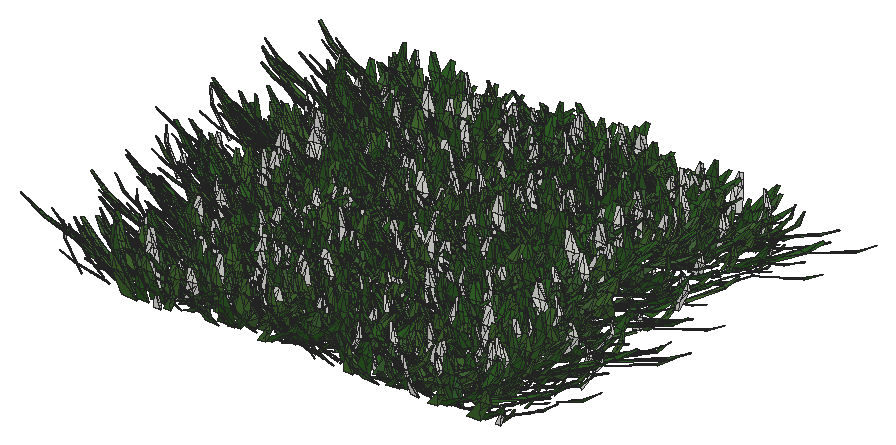
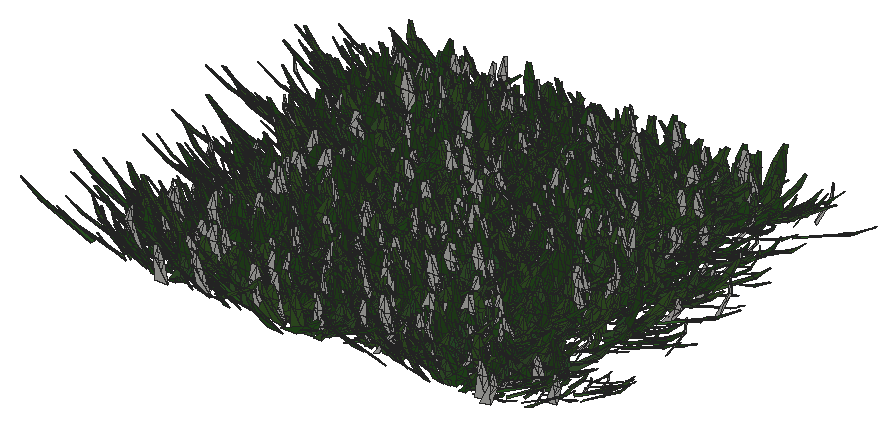
# SketchUp Ruby script. Lengths in inches.
U = 1.inch
M = Sketchup.active_model
def pt(a) = Geom::Point3d.new(a.map { |v| v * U })
def face(e, loops, mat)
  f = e.add_face(loops[0].map { |a| pt(a) })
  loops[1..].each { |l| e.add_face(l.map { |a| pt(a) }).erase! }
  f.material = f.back_material = mat if mat
  f
end
# faces: each face lists its corners as indices into pts; further lists are holes
def faces(e, pts, list, mat = nil) = list.each { |f| face(e, (f[0].is_a?(Array) ? f : [f]).map { |l| l.map { |i| pts[i] } }, mat) }
# xy, xz, yz: faces in a plane at the given z, y or x. An outline is a flat list of corners, or four numbers for a rectangle; further outlines are holes
def ring(l) = l.size == 4 ? [[l[0], l[1]], [l[2], l[1]], [l[2], l[3]], [l[0], l[3]]] : l.each_slice(2).to_a
def flat(e, list, mat, &to3) = list.each { |f| face(e, (f[0].is_a?(Array) ? f : [f]).map { |l| ring(l).map { |u, v| to3.(u, v) } }, mat) }
def xy(e, z, list, mat = nil) = flat(e, list, mat) { |x, y| [x, y, z] }
def xz(e, y, list, mat = nil) = flat(e, list, mat) { |x, z| [x, y, z] }
def yz(e, x, list, mat = nil) = flat(e, list, mat) { |y, z| [x, y, z] }
def lines(e, pts, list) = list.each { |a, b| e.add_line(pt(pts[a]), pt(pts[b])) }
# prism: a flat outline (further loops are holes) pulled along v
def prism(e, loops, v, mat = nil)
  f = face(e, loops, mat); d = Geom::Vector3d.new(v.map { |x| x * U })
  f.pushpull(f.normal.samedirection?(d) ? d.length : -d.length)
end
def box(e, o, s, mat = nil) = prism(e, [[o, [o[0] + s[0], o[1], o[2]], [o[0] + s[0], o[1] + s[1], o[2]], [o[0], o[1] + s[1], o[2]]]], [0, 0, s[2]], mat)
def at(x, y, z, deg = 0) = Geom::Transformation.translation(pt([x, y, z])) * Geom::Transformation.rotation(ORIGIN, Z_AXIS, deg.degrees)
def axes(o, x, y, z) = Geom::Transformation.new([*x, 0, *y, 0, *z, 0, *pt(o).to_a, 1])
def part(name) = M.definitions.add(name)
# library, detail: a bought-in or finely detailed component or shape, given as its bounding box
def library(name, o, s) = part(name).tap { |d| box(d.entities, o, s) }
def detail(e, o, s) = box(e.add_group.entities, o, s)
def put(e, d, t, mat = nil) = e.add_instance(d, t).tap { |i| i.material = mat if mat }
def group(e, t, mat = nil) = e.add_group.tap { |g| g.transformation = t; g.material = mat if mat }.entities
root = M.entities
M.materials.add("Material10").color = [48, 100, 38]
M.materials.add("Material3").color = [68, 110, 58]
M.materials.add("Material4").color = [48, 90, 38]
M.materials.add("Material5").color = [68, 110, 48]
M.materials.add("Material6").color = [48, 90, 48]
M.materials.add("Material7").color = [58, 110, 58]
M.materials.add("Material8").color = [58, 90, 38]
M.materials.add("Material9").color = [68, 100, 58]
c1 = part("grass00")
p = [[-0.6875,0.15,0],[-0.56,0.08,5.52],[-0.04,0.03,2.76],[0.48,-0.02,0],[0.35,-0.02,5.52],[-0.1,-0.14,5.52],
  [-0.12,0.65,8.37],[-0.42,0.65,8.37]]
faces(c1.entities,p,[[0,1,2,3],[3,2,4],[1,5,2],[5,4,2],[1,6,5],[4,5,6],[7,6,1]])
c2 = part("Group16\#1")
put(c2.entities,c1,axes([1.44,-0.61,-0.01],[0.05352,0.12609,0],[-0.10704,0.04543,0.07239],[0.06664,-0.02828,0.11628]),"Material6")
put(c2.entities,c1,axes([0.76,-0.15,-0.01],[0.04676,0.24062,0],[-0.23162,0.04501,0.06642],[0.0652,-0.01267,0.23595]),"Material3")
put(c2.entities,c1,axes([0.79,0.01,-0.01],[-0.00606,0.34651,0],[-0.34381,-0.00602,0.0432],[0.04319,0.00076,0.34386]))
put(c2.entities,c1,axes([1,0.23,-0.01],[-0.07192,0.31144,0],[-0.28722,-0.06632,0.1236],[0.12043,0.02781,0.29478]),"Material5")
put(c2.entities,c1,axes([1.66,0.77,-0.01],[-0.13828,0.29651,0],[-0.21551,-0.1005,0.22471],[0.20365,0.09498,0.23779]),"Material10")
put(c2.entities,c1,axes([0.6875,0.52,-0.01],[-0.18126,0.24051,0],[-0.22746,-0.17142,0.09788],[0.07817,0.05891,0.28481]),"Material5")
put(c2.entities,c1,axes([0.68,0.78,-0.01],[-0.215,0.18688,0],[-0.12385,-0.14248,0.21334],[0.13995,0.16101,0.18878]),"Material3")
put(c2.entities,c1,axes([0.56,1,-0.01],[-0.13756,0.07624,0],[-0.06159,-0.11112,0.0927],[0.04494,0.08108,0.12705]),"Material5")
put(c2.entities,c1,axes([0.2,0.64,-0.01],[-0.23729,0.07254,0],[-0.05711,-0.18681,0.153],[0.04473,0.14632,0.19535]),"Material10")
put(c2.entities,c1,axes([0.0625,0.72,-0.01],[-0.28874,0.02525,0],[-0.02179,-0.24916,0.14647],[0.01276,0.14591,0.25012]),"Material3")
put(c2.entities,c1,axes([-0.08,0.62,-0.01],[-0.34089,-0.04187,0],[0.03255,-0.26504,0.216],[-0.02633,0.21439,0.26703]),"Material10")
put(c2.entities,c1,axes([-0.34,0.98,-0.01],[-0.14314,-0.0493,0],[0.04397,-0.12769,0.06843],[-0.02228,0.0647,0.13505]),"Material10")
put(c2.entities,c1,axes([-0.87,1.45,-0.01],[-0.23488,-0.14114,0],[0.13761,-0.22901,0.06087],[-0.03135,0.05217,0.26717]))
put(c2.entities,c1,axes([-0.72,0.77,-0.01],[-0.14208,-0.13251,0],[0.07209,-0.0773,0.16301],[-0.11118,0.11922,0.1057]),"Material10")
put(c2.entities,c1,axes([-0.62,0.43,-0.01],[-0.14845,-0.21203,0],[0.18654,-0.13061,0.12304],[-0.10079,0.07057,0.22772]),"Material3")
put(c2.entities,c1,axes([-0.68,0.29,-0.01],[-0.13639,-0.32136,0],[0.31723,-0.13464,0.05579],[-0.05136,0.0218,0.34462]),"Material4")
put(c2.entities,c1,axes([-0.64,0.125,-0.01],[-0.0458,-0.23569,0],[0.22124,-0.043,0.08276],[-0.08124,0.01579,0.22538]),"Material7")
put(c2.entities,c1,axes([-1.6,-0.03,-0.01],[0.00576,-0.32897,0],[0.27526,0.00482,0.18018],[-0.18015,-0.00315,0.2753]),"Material5")
put(c2.entities,c1,axes([-1.36,-0.31,-0.01],[0.05718,-0.24765,0],[0.18172,0.04196,0.17267],[-0.16825,-0.03885,0.1865]),"Material10")
put(c2.entities,c1,axes([-1.54,-0.72,-0.01],[0.06537,-0.14017,0],[0.13555,0.06321,0.03939],[-0.0357,-0.01665,0.14956]))
put(c2.entities,c1,axes([-1.19,-0.9,-0.01],[0.09597,-0.12735,0],[0.11214,0.08451,0.07557],[-0.06035,-0.04548,0.14042]),"Material9")
put(c2.entities,c1,axes([-0.47,-0.54,-0.01],[0.11588,-0.10072,0],[0.0618,0.0711,0.12124],[-0.07953,-0.0915,0.0942]))
put(c2.entities,c1,axes([-0.47,-0.84,-0.01],[0.11927,-0.0661,0],[0.06603,0.11913,0.00646],[-0.00313,-0.00565,0.13621]),"Material5")
put(c2.entities,c1,axes([-0.38,-1.24,-0.01],[0.28037,-0.08571,0],[0.0618,0.20215,0.20315],[-0.05939,-0.19428,0.21139]),"Material9")
put(c2.entities,c1,axes([-0.06,-0.66,-0.01],[0.22719,-0.01987,0],[0.01247,0.14255,0.17758],[-0.01547,-0.17691,0.1431]),"Material8")
put(c2.entities,c1,axes([0.11,-0.89,-0.01],[0.14882,0.01828,0],[-0.01058,0.08611,0.12229],[0.01491,-0.12138,0.08676]),"Material6")
put(c2.entities,c1,axes([0.25,-0.72,-0.01],[0.20481,0.07053,0],[-0.06206,0.18022,0.10291],[0.03351,-0.0973,0.1906]),"Material6")
put(c2.entities,c1,axes([0.85,-1.42,-0.01],[0.16481,0.09904,0],[-0.09472,0.15762,0.05616],[0.02893,-0.04814,0.18389]),"Material5")
put(c2.entities,c1,axes([1.01,-1.09,-0.01],[0.21858,0.20385,0],[-0.17495,0.1876,0.15339],[0.10462,-0.11218,0.25652]),"Material10")
put(c2.entities,c1,axes([1.01,-0.71,-0.01],[0.08733,0.12473,0],[-0.06445,0.04512,0.13037],[0.1068,-0.07477,0.07867]),"Material6")
c3 = part("Group15\#1")
put(c3.entities,c2,at(0,0,0))
c4 = part("3darcstudiotree_grass00\#1")
put(c4.entities,c3,at(0,0,0))
put(root,c4,axes([1060.01,968.44,0],[3.81538,0.13844,0],[-0.69714,1.20077,-0.0224],[-0.01503,0.02589,1.41716]))
put(root,c4,axes([1060.61,966.34,0],[3.87873,-0.1816,0],[0.87965,1.17427,-0.05648],[0.04872,0.06503,1.39957]))
put(root,c4,axes([1060.62,949.85,0],[2.2908,0.71526,0],[-3.14647,0.62983,-0.01526],[-0.09231,0.01848,1.9517]))
put(root,c4,axes([1060.87,957.6,0],[1.88546,0.82083,0],[-4.0871,0.58676,-0.0451],[-0.25686,0.03688,1.93445]))
put(root,c4,axes([1064,960.65,0],[-3.85189,-0.43073,0],[1.56903,-0.87695,-0.00732],[0.02092,-0.01169,1.68082]))
put(root,c4,axes([1063.95,942.66,0],[-1.50152,-0.9142,0],[4.09435,-0.4203,-0.04381],[0.2556,-0.02624,1.74465]))
put(root,c4,axes([1064.63,951.69,0],[-0.92252,-0.87304,0],[4.75689,-0.31416,-0.01354],[0.0811,-0.00536,1.90468]))
put(root,c4,axes([1063.46,971.5,0],[4.15823,-0.14638,0],[0.56684,1.00637,-0.04526],[0.04452,0.07905,1.7925]))
put(root,c4,axes([1065.13,934.82,0],[-1.25145,-1.20565,0],[3.82205,-0.24795,-0.03225],[0.20024,-0.01299,1.58326]))
put(root,c4,axes([1064.48,958.88,0],[-3.10495,0.65805,0],[-2.73218,-0.80572,-0.0209],[-0.07578,-0.02235,1.48072]))
put(root,c4,axes([1063.8,933.42,0],[0.14781,1.06815,0],[-4.11052,0.03555,-0.02489],[-0.18669,0.00161,1.9295]))
put(root,c4,axes([1063.73,948.06,0],[4.00072,0.7254,0],[-2.30793,0.79554,-0.01189],[-0.04272,0.01473,1.50367]))
put(root,c4,axes([1064.75,958.07,0],[-2.74027,0.72148,0],[-3.68495,-0.87475,-0.01749],[-0.07151,-0.01698,1.7911]))
put(root,c4,axes([1065.1,945.05,0],[-2.75544,0.79472,0],[-3.06036,-0.66317,-0.04719],[-0.18345,-0.03975,1.30223]))
put(root,c4,axes([1065.82,968.08,0],[1.11217,-0.96649,0],[4.59277,0.33032,-0.0144],[0.08373,0.00602,1.80693]))
put(root,c4,axes([1065.92,954.83,0],[-4.93169,0.08818,0],[-0.36054,-1.26027,-0.06114],[-0.024,-0.08388,1.73764]))
put(root,c4,axes([1064.06,952.93,0],[3.76135,0.71254,0],[-2.83931,0.93675,-0.0181],[-0.05013,0.01654,1.34745]))
put(root,c4,axes([1064.44,964.01,0],[0.92537,1.06658,0],[-3.52867,0.19134,-0.00976],[-0.0687,0.00373,1.62508]))
put(root,c4,axes([1065.98,936.2,0],[-4.59841,0.23812,0],[-1.05246,-1.27026,-0.05761],[-0.06188,-0.07469,1.71741]))
put(root,c4,axes([1065.1,950.4375,0],[3.52248,-0.74116,0],[2.46477,0.73213,-0.04982],[0.1917,0.05694,1.4295]))
put(root,c4,axes([1065.57,956.52,0],[-2.75303,1.02553,0],[-3.67007,-0.61577,-0.03945],[-0.19029,-0.03193,1.6047]))
put(root,c4,axes([1066.68,938.42,0],[0.13208,-1.10378,0],[4.58182,0.03427,-0.01737],[0.09381,0.0007,1.54781]))
put(root,c4,axes([1065.45,972.2,0],[3.94098,0.32291,0],[-1.45311,1.10842,-0.04711],[-0.07836,0.05977,1.55738]))
put(root,c4,axes([1067.3,946.65,0],[-4.05461,-0.34542,0],[1.65205,-1.21201,-0.06303],[0.10229,-0.07504,1.61067]))
put(root,c4,axes([1066.19,939.92,0],[-0.37634,1.08622,0],[-3.78806,-0.08203,-0.04948],[-0.29529,-0.00639,1.42361]))
put(root,c4,axes([1065.71,943.77,0],[1.93194,0.81354,0],[-3.84457,0.57061,-0.05173],[-0.21974,0.03261,1.38038]))
put(root,c4,axes([1067.08,969.37,0],[2.66553,-1.02305,0],[4.32772,0.70474,-0.04483],[0.19345,0.0315,1.66248]))
put(root,c4,axes([1067.12,966.35,0],[-4.37352,0.6514,0],[-2.31701,-0.97227,-0.00882],[-0.02275,-0.00955,1.42641]))
put(root,c4,axes([1066.53,940.98,0],[4.99102,-0.01521,0],[0.04604,0.94447,-0.04731],[0.00388,0.07956,1.58849]))
put(root,c4,axes([1067.67,964.9375,0],[3.89455,0.04164,0],[-0.19515,1.14083,-0.05798],[-0.01392,0.08139,1.60438]))
put(root,c4,axes([1067.37,961.9,0],[2.5974,0.75785,0],[-3.87592,0.83025,-0.05975],[-0.19783,0.04238,1.3909]))
put(root,c4,axes([1070.43,954.99,0],[-4.50466,-0.2627,0],[0.84333,-0.90382,-0.01564],[0.02098,-0.02248,1.3694]))
put(root,c4,axes([1071.07,951.4,0],[-4.10148,-0.37644,0],[1.4137,-0.96268,-0.02574],[0.04791,-0.03263,1.38465]))
put(root,c4,axes([1070.94,948.83,0],[-4.28392,0.00118,0],[-0.00439,-0.99985,-0.04481],[-0.00034,-0.07634,1.70362]))
put(root,c4,axes([1071.18,963.31,0],[-4.02766,-0.18324,0],[0.7232,-0.9935,-0.02729],[0.03622,-0.04975,1.8715]))
put(root,c4,axes([1071.04,965.58,0],[1.16692,-1.18724,0],[4.2577,0.26155,-0.05295],[0.37072,0.02277,1.97565]))
put(root,c4,axes([1071.97,959.11,0],[-4.78558,-0.30533,0],[0.89073,-0.87254,-0.00096],[0.00166,-0.00163,1.58162]))
put(root,c4,axes([1071.53,962.42,0],[1.62332,-1.0011,0],[4.766,0.48301,-0.03495],[0.18538,0.01879,1.83937]))
put(root,c4,axes([1072.25,941.04,0],[-4.37321,-0.34262,0],[1.17174,-0.93477,-0.00157],[0.00264,-0.00211,1.37913]))
put(root,c4,axes([1071.75,960.11,0],[0.5215,-1.25098,0],[3.70627,0.09657,-0.02929],[0.19507,0.00508,1.55926]))
put(root,c4,axes([1072.1875,935.32,0],[-1.52927,-0.99373,0],[4.10162,-0.3945,-0.0371],[0.24735,-0.02379,1.96201]))
put(root,c4,axes([1071.96,970.28,0],[-2.5925,0.65112,0],[-2.57682,-0.64124,-0.04592],[-0.2048,-0.05096,1.42994]))
put(root,c4,axes([1070.98,952.76,0],[2.46517,0.89808,0],[-3.36918,0.57801,-0.0512],[-0.22975,0.03942,1.38975]))
put(root,c4,axes([1071.74,946.98,0],[-1.95791,0.95694,0],[-3.80128,-0.48609,-0.05082],[-0.22925,-0.02932,1.35221]))
put(root,c4,axes([1070.95,945.78,0],[3.4935,0.9356,0],[-3.37227,0.78699,-0.04297],[-0.21601,0.05041,1.98261]))
put(root,c4,axes([1072.5625,949.54,0],[-3.83195,0.74101,0],[-2.84787,-0.92045,-0.05181],[-0.15821,-0.05114,1.45196]))
put(root,c4,axes([1072.74,968.71,0],[1.45199,-1.1226,0],[3.82197,0.30896,-0.02554],[0.13596,0.01099,1.40467]))
put(root,c4,axes([1072.63,958.05,0],[0.21484,-1.19151,0],[3.62833,0.04089,-0.03915],[0.33615,0.00379,1.95085]))
put(root,c4,axes([1072.78,944.46,0],[-4.05301,0.5506,0],[-2.43371,-1.11967,-0.04664],[-0.11424,-0.05256,1.63424]))
put(root,c4,axes([1072.64,956.5625,0],[2.22271,-0.98365,0],[3.97274,0.56106,-0.05349],[0.32137,0.04539,1.96798]))
put(root,c4,axes([1071.54,971.14,0],[2.83397,0.77998,0],[-3.02687,0.68736,-0.01914],[-0.0787,0.01787,1.41957]))
put(root,c4,axes([1071.36,936.42,0],[1.59207,1.04289,0],[-4.49774,0.42914,-0.00597],[-0.03376,0.00322,1.82255]))
put(root,c4,axes([1071.99,933.84,0],[3.98575,0.27966,0],[-0.97946,0.87245,-0.00495],[-0.0082,0.00731,1.38942]))
put(root,c4,axes([1072.27,966.23,0],[4.21135,-0.01817,0],[0.08044,1.16521,-0.0287],[0.00337,0.04884,1.98369]))
put(root,c4,axes([1072.75,939.42,0],[-2.028,0.74895,0],[-3.60661,-0.61038,-0.00267],[-0.01315,-0.00223,1.62102]))
put(root,c4,axes([1073.56,942.1,0],[3.07423,-0.81379,0],[3.32943,0.78609,-0.05261],[0.18555,0.04381,1.38839]))
put(root,c4,axes([1072.82,937.74,0],[3.5941,0.56914,0],[-2.69156,1.06232,-0.01012],[-0.02733,0.01079,1.58691]))
put(root,c4,axes([1075.71,940.98,0],[-0.91152,-0.89442,0],[3.63132,-0.23129,-0.03395],[0.21582,-0.01375,1.53644]))
put(root,c4,axes([1076.09,943.5,0],[-0.47866,-0.98426,0],[5.08014,-0.15441,-0.04217],[0.1851,-0.00563,1.41426]))
put(root,c4,axes([1076.28,954.85,0],[-3.99249,-0.2843,0],[1.19862,-1.05202,-0.03955],[0.07734,-0.06788,1.95202]))
put(root,c4,axes([1075.46,947.38,0],[4.25304,-0.27501,0],[1.24647,1.20478,-0.04841],[0.06924,0.06692,1.77682]))
put(root,c4,axes([1075.74,959.03,0],[3.55406,-0.41539,0],[2.08359,1.1142,-0.04906],[0.12364,0.06612,1.82977]))
put(root,c4,axes([1077.04,936.3125,0],[-0.93715,-1.08339,0],[4.95712,-0.268,-0.05631],[0.2396,-0.01295,1.37991]))
put(root,c4,axes([1077.33,945.36,0],[-3.14134,-0.50366,0],[2.13341,-0.83163,-0.01822],[0.06361,-0.0248,1.59761]))
put(root,c4,axes([1077.07,938.9375,0],[-3.94175,0.51659,0],[-1.67373,-0.7982,-0.02232],[-0.07314,-0.03488,1.59039]))
put(root,c4,axes([1075.57,948.76,0],[1.62757,0.88807,0],[-4.34169,0.49732,-0.00338],[-0.01586,0.00182,1.53978]))
put(root,c4,axes([1076.37,968.32,0],[4.57989,-0.16103,0],[0.69599,1.23718,-0.01318],[0.01167,0.02075,1.98636]))
put(root,c4,axes([1077.74,951.39,0],[1.79397,-1.16047,0],[4.15779,0.40172,-0.011],[0.05477,0.00529,1.48653]))
put(root,c4,axes([1078.22,935.36,0],[-3.09464,-0.54466,0],[2.39537,-0.85062,-0.03828],[0.16794,-0.05964,1.98208]))
put(root,c4,axes([1076.89,957.33,0],[0.16957,1.15455,0],[-4.45398,0.04088,-0.05084],[-0.31058,0.00285,1.70302]))
put(root,c4,axes([1077.39,961.91,0],[3.46351,-0.6215,0],[2.10035,0.73155,-0.02763],[0.09487,0.03304,1.3256]))
put(root,c4,axes([1078.47,956.5,0],[-1.3865,-0.85758,0],[4.31936,-0.43646,-0.05241],[0.27908,-0.0282,1.67241]))
put(root,c4,axes([1078.63,965.44,0],[-4.39937,-0.11992,0],[0.44419,-1.01847,-0.05296],[0.03633,-0.08329,1.62079]))
put(root,c4,axes([1079.33,938.4,0],[-1.76031,-0.79386,0],[4.32977,-0.60005,-0.00731],[0.04086,-0.00566,1.97847]))
put(root,c4,axes([1079.32,969.55,0],[-2.83446,-0.91757,0],[3.42874,-0.66198,-0.00917],[0.043,-0.0083,1.60374]))
put(root,c4,axes([1078.99,963.69,0],[-0.96511,-1.1714,0],[4.02104,-0.20706,-0.02826],[0.17189,-0.00885,1.59374]))
put(root,c4,axes([1078.17,966.53,0],[-2.51846,0.95711,0],[-4.14801,-0.68217,-0.04701],[-0.20561,-0.03381,1.62457]))
put(root,c4,axes([1079.36,950.15,0],[-3.64421,0.19897,0],[-0.82865,-0.94858,-0.01018],[-0.01217,-0.01393,1.35975]))
put(root,c4,axes([1078.29,942.02,0],[4.36646,0.14498,0],[-0.67462,1.26988,-0.05242],[-0.04036,0.07596,1.87281]))
put(root,c4,axes([1079.25,971.55,0],[3.61828,-0.3087,0],[1.22458,0.89709,-0.02189],[0.0555,0.04066,1.86062]))
put(root,c4,axes([1079.38,952.58,0],[-0.33218,0.92371,0],[-3.73108,-0.08386,-0.0349],[-0.21038,-0.00473,1.41691]))
put(root,c4,axes([1079.45,961.08,0],[3.6543,-0.06929,0],[0.34871,1.14948,-0.06006],[0.02412,0.07952,1.53056]))
put(root,c4,axes([1079.95,972.55,0],[2.4776,1.07425,0],[-3.76626,0.5429,-0.02249],[-0.11657,0.0168,1.62577]))
put(root,c4,axes([1081.93,961,0],[1.28704,-1.14477,0],[4.41434,0.31018,-0.04021],[0.23445,0.01647,1.73573]))
put(root,c4,axes([1082.32,966.49,0],[-3.66743,0.44114,0],[-1.9663,-1.02167,-0.05656],[-0.13362,-0.06943,1.54444]))
put(root,c4,axes([1082.53,971.34,0],[-3.63818,0.44085,0],[-1.59896,-0.82474,-0.04774],[-0.15109,-0.07793,1.66266]))
put(root,c4,axes([1082.95,936.69,0],[-3.07397,-0.63014,0],[2.5257,-0.77005,-0.04795],[0.16981,-0.05177,1.39039]))
put(root,c4,axes([1081.92,938.9,0],[3.59272,-0.42375,0],[1.98946,1.05421,-0.02435],[0.06043,0.03202,1.69455]))
put(root,c4,axes([1083.11,964.9,0],[-2.26382,-1.02381,0],[3.25832,-0.45029,-0.04183],[0.23401,-0.03234,1.48723]))
put(root,c4,axes([1083.21,949.46,0],[-1.57651,-1.12747,0],[4.0703,-0.35571,-0.03865],[0.26242,-0.02293,1.9383]))
put(root,c4,axes([1081.78,963.1,0],[1.17301,1.14331,0],[-4.44463,0.28501,-0.04684],[-0.2246,0.0144,1.41954]))
put(root,c4,axes([1081.97,955.125,0],[4.31123,0.22817,0],[-0.83721,0.9887,-0.03259],[-0.04316,0.05097,1.61556]))
put(root,c4,axes([1081.96,969.97,0],[3.06774,1.03902,0],[-3.08129,0.5686,-0.03251],[-0.17928,0.03308,1.64081]))
put(root,c4,axes([1084.33,962.35,0],[-2.08621,-0.85991,0],[3.58173,-0.54309,-0.01057],[0.06396,-0.0097,1.85267]))
put(root,c4,axes([1083.97,951.53,0],[-4.18093,0.10999,0],[-0.54376,-1.29184,-0.00853],[-0.00476,-0.01131,1.7318]))
put(root,c4,axes([1084.74,941.4375,0],[-3.42299,-0.52038,0],[2.6642,-1.0953,-0.06276],[0.1523,-0.06261,1.49667]))
put(root,c4,axes([1082.96,938.17,0],[3.25907,0.53746,0],[-2.27195,0.86105,-0.03997],[-0.15705,0.05952,1.84008]))
put(root,c4,axes([1084.98,943.54,0],[-2.53551,-0.66282,0],[3.06498,-0.73279,-0.03327],[0.11879,-0.0284,1.30962]))
put(root,c4,axes([1083.78,959.47,0],[-1.21767,0.90066,0],[-3.71776,-0.31415,-0.04196],[-0.263,-0.02222,1.62262]))
put(root,c4,axes([1085.06,946.81,0],[-4.32463,-0.20055,0],[0.81802,-1.10246,-0.00704],[0.00853,-0.0115,1.86241]))
put(root,c4,axes([1083.54,955.625,0],[-0.94156,1.16657,0],[-3.85079,-0.19425,-0.00527],[-0.04036,-0.00204,1.91768]))
put(root,c4,axes([1083.86,953.26,0],[-1.89095,0.77708,0],[-4.00997,-0.60986,-0.02284],[-0.10942,-0.01664,1.64481]))
put(root,c4,axes([1084.66,967.76,0],[-3.52622,0.53949,0],[-2.34194,-0.95671,-0.04749],[-0.11586,-0.04733,1.3106]))
put(root,c4,axes([1084.31,941.9375,0],[-0.72165,1.07172,0],[-4.22626,-0.17786,-0.04712],[-0.23093,-0.00972,1.33133]))
put(root,c4,axes([1083.87,945.625,0],[1.97727,0.77994,0],[-4.30152,0.68157,-0.01772],[-0.06482,0.01027,1.37883]))
put(root,c4,axes([1085.28,934.88,0],[3.9848,-0.55599,0],[2.03989,0.91374,-0.03495],[0.12387,0.05549,1.90256]))
put(root,c4,axes([1085.09,972.32,0],[-0.75919,1.1846,0],[-4.72482,-0.18925,-0.01053],[-0.05452,-0.00218,1.56894]))
put(root,c4,axes([1085.86,948.05,0],[-2.69032,0.86465,0],[-3.81847,-0.74256,-0.01031],[-0.04487,-0.00873,1.66779]))
put(root,c4,axes([1085.23,957.34,0],[4.37586,0.6715,0],[-2.05906,0.83863,-0.0354],[-0.14622,0.05955,1.94218]))
put(root,c4,axes([1087.94,971.52,0],[3.53194,-0.86434,0],[3.34252,0.85365,-0.00616],[0.02391,0.00611,1.65812]))
put(root,c4,axes([1087.54,942.53,0],[-1.22084,1.17012,0],[-4.22614,-0.27558,-0.04083],[-0.27889,-0.01819,1.92702]))
put(root,c4,axes([1088.77,956.5625,0],[2.5391,-0.86121,0],[4.09888,0.75529,-0.00987],[0.04755,0.00876,1.9048]))
put(root,c4,axes([1088.11,952.86,0],[4.20042,-0.44882,0],[1.64886,0.96446,-0.01454],[0.02841,0.01662,1.30369]))
put(root,c4,axes([1089.15,967.04,0],[-3.69839,0.06543,0],[-0.3293,-1.16339,-0.01026],[-0.00422,-0.01493,1.70108]))
put(root,c4,axes([1088.65,962.53,0],[2.45158,-0.94892,0],[4.05066,0.65407,-0.0579],[0.29835,0.04817,1.84885]))
put(root,c4,axes([1089.03,951.41,0],[-3.62062,0.56511,0],[-2.64905,-1.06077,-0.02972],[-0.08176,-0.03274,1.62371]))
put(root,c4,axes([1088.37,960.49,0],[4.94305,-0.26827,0],[1.01972,1.17431,-0.03342],[0.04517,0.05201,1.91382]))
put(root,c4,axes([1088.93,934.53,0],[5.06338,0.28931,0],[-0.91613,1.00212,-0.00333],[-0.00395,0.00432,1.36941]))
put(root,c4,axes([1090.74,939.61,0],[-3.99538,-0.04123,0],[0.20618,-1.24865,-0.05407],[0.01202,-0.0728,1.68402]))
put(root,c4,axes([1089.16,936.07,0],[2.5961,0.65731,0],[-3.59247,0.8868,-0.04002],[-0.16483,0.04069,1.82631]))
put(root,c4,axes([1090.21,949.96,0],[-3.34956,0.74843,0],[-3.0511,-0.85344,-0.02716],[-0.08391,-0.02347,1.32671]))
put(root,c4,axes([1091.4375,948.29,0],[-2.33326,-1.15563,0],[4.19034,-0.52878,-0.02075],[0.1057,-0.01334,1.67433]))
put(root,c4,axes([1090.15,967.84,0],[3.85684,-0.72833,0],[2.27457,0.7528,-0.01203],[0.05895,0.01951,1.91781]))
put(root,c4,axes([1091.38,940.99,0],[-4.81633,-0.15482,0],[0.50253,-0.97708,-0.03967],[0.03663,-0.07121,1.78282]))
put(root,c4,axes([1091.26,959.49,0],[-4.3189,0.23802,0],[-0.87038,-0.98708,-0.01188],[-0.02021,-0.02292,1.99665]))
put(root,c4,axes([1090.68,954.46,0],[3.261,-0.91173,0],[3.2122,0.71807,-0.03435],[0.17461,0.03903,1.83666]))
put(root,c4,axes([1089.98,963.71,0],[0.9409,1.10722,0],[-4.02636,0.21385,-0.01067],[-0.07425,0.00394,1.82972]))
put(root,c4,axes([1091.71,945.78,0],[-4.23033,0.08475,0],[-0.4056,-1.2654,-0.02116],[-0.00955,-0.02979,1.79229]))
put(root,c4,axes([1091.26,964.74,0],[3.52347,0.24028,0],[-1.10282,1.01075,-0.00322],[-0.00644,0.0059,1.99197]))
put(root,c4,axes([1091.14,957.12,0],[1.43969,0.92574,0],[-4.67724,0.45462,-0.01993],[-0.11798,0.01147,1.99239]))
put(root,c4,axes([1091.79,947.31,0],[5.05994,-0.2516,0],[1.00622,1.26478,-0.02703],[0.02801,0.03521,1.71263]))
put(root,c4,axes([1091.67,943.39,0],[4.82559,0.20741,0],[-0.80452,1.16986,-0.00744],[-0.0078,0.01134,1.83611]))
put(root,c4,axes([1091.93,969.4,0],[0.8534,1.21084,0],[-4.69984,0.20703,-0.04576],[-0.24908,0.01097,1.64855]))
put(root,c4,axes([1091.75,937.97,0],[3.19918,0.93159,0],[-3.22991,0.69324,-0.03135],[-0.15607,0.0335,1.74596]))
put(root,c4,axes([1093.6875,948.27,0],[-4.78772,-0.06379,0],[0.24177,-1.13418,-0.04256],[0.01334,-0.06257,1.67228]))
put(root,c4,axes([1094.38,942.55,0],[-0.71675,-1.13994,0],[5.03401,-0.19782,-0.0381],[0.22843,-0.00898,1.93318]))
put(root,c4,axes([1094.3,959.13,0],[-3.55446,-0.53666,0],[1.86548,-0.77223,-0.04514],[0.17034,-0.07051,1.64638]))
put(root,c4,axes([1094.3,964.7,0],[-3.57017,-0.151,0],[0.63334,-0.9359,-0.02254],[0.02209,-0.03264,1.39425]))
put(root,c4,axes([1093.72,939.07,0],[3.4593,-0.56145,0],[2.1047,0.8105,-0.02789],[0.10781,0.04152,1.71527]))
put(root,c4,axes([1094.625,940.45,0],[-3.94355,0.22015,0],[-0.99731,-1.11654,-0.00123],[-0.00186,-0.00209,1.99006]))
put(root,c4,axes([1094.17,968.2,0],[3.30228,-0.99674,0],[2.91611,0.60383,-0.04892],[0.25342,0.05247,1.59182]))
put(root,c4,axes([1093.69,967.05,0],[4.61986,0.38616,0],[-1.27131,0.9506,-0.01696],[-0.03888,0.02907,1.81122]))
put(root,c4,axes([1094.89,971.08,0],[-2.0103,0.88344,0],[-3.56839,-0.5075,-0.04597],[-0.20616,-0.02932,1.32398]))
put(root,c4,axes([1094.69,972.63,0],[3.96671,-0.47551,0],[1.66213,0.8666,-0.03326],[0.09836,0.05128,1.64345]))
put(root,c4,axes([1094.49,937.73,0],[2.08308,0.83791,0],[-3.29361,0.51175,-0.00184],[-0.01033,0.00161,1.60144]))
put(root,c4,axes([1094.95,954.87,0],[-1.06068,0.91839,0],[-4.56893,-0.3298,-0.01983],[-0.09265,-0.00669,1.44555]))
put(root,c4,axes([1095.49,934.97,0],[-1.97754,0.85348,0],[-3.2966,-0.47739,-0.02138],[-0.12695,-0.01838,1.63406]))
put(root,c4,axes([1095.48,947.32,0],[-1.2265,1.05965,0],[-4.78236,-0.34596,-0.06381],[-0.32881,-0.02379,1.66913]))
